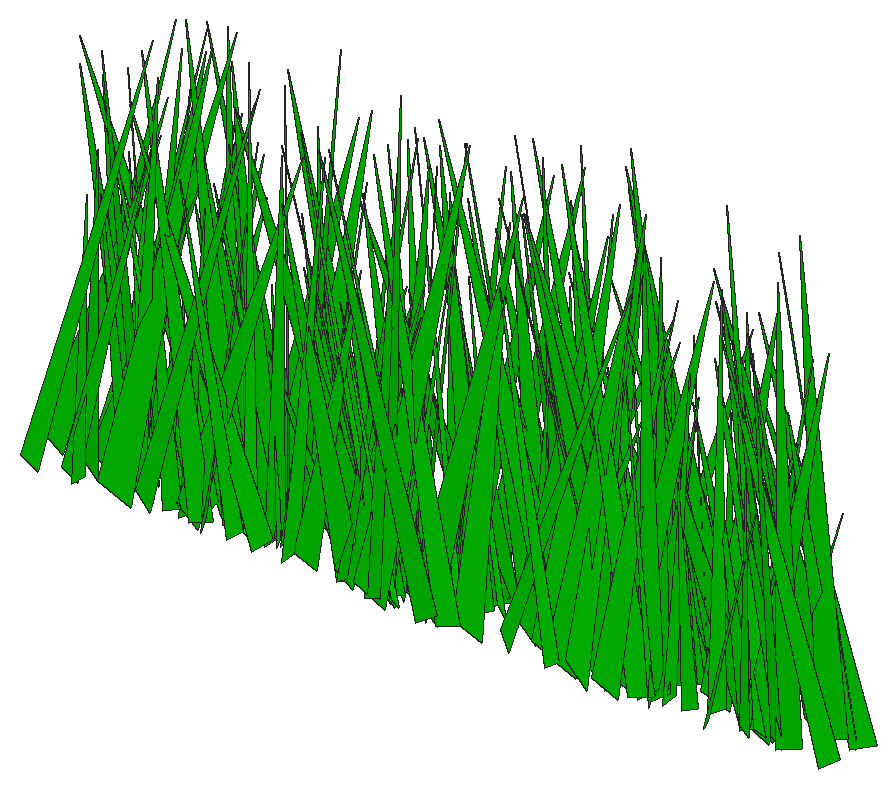
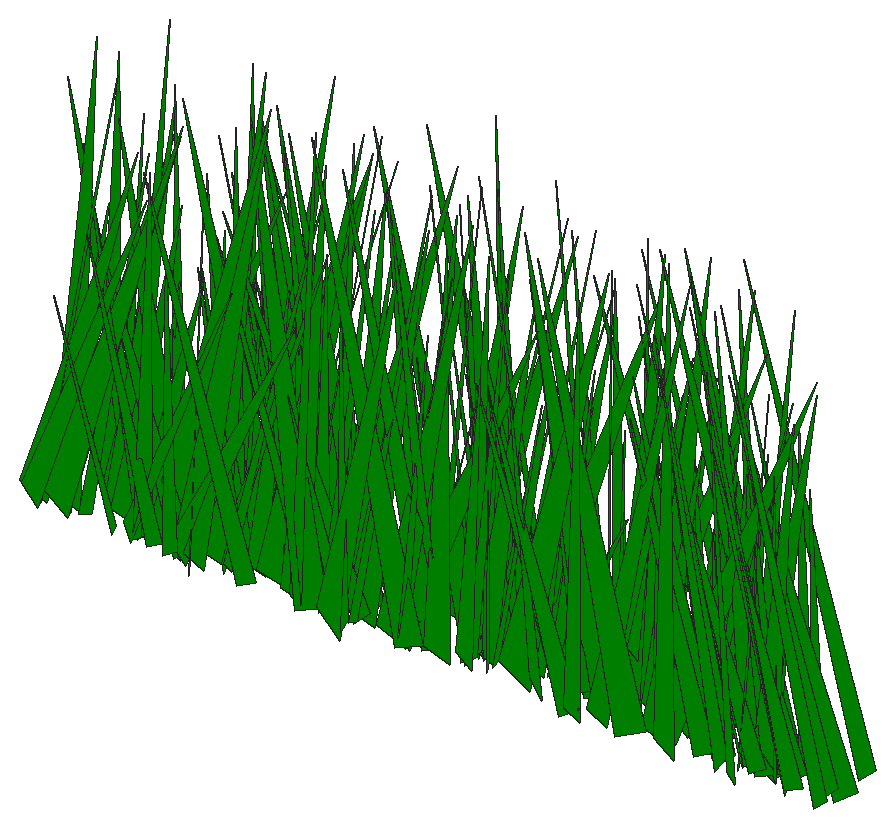
# SketchUp Ruby script. Lengths in inches.
U = 1.inch
M = Sketchup.active_model
def pt(a) = Geom::Point3d.new(a.map { |v| v * U })
def face(e, loops, mat)
  f = e.add_face(loops[0].map { |a| pt(a) })
  loops[1..].each { |l| e.add_face(l.map { |a| pt(a) }).erase! }
  f.material = f.back_material = mat if mat
  f
end
# faces: each face lists its corners as indices into pts; further lists are holes
def faces(e, pts, list, mat = nil) = list.each { |f| face(e, (f[0].is_a?(Array) ? f : [f]).map { |l| l.map { |i| pts[i] } }, mat) }
# xy, xz, yz: faces in a plane at the given z, y or x. An outline is a flat list of corners, or four numbers for a rectangle; further outlines are holes
def ring(l) = l.size == 4 ? [[l[0], l[1]], [l[2], l[1]], [l[2], l[3]], [l[0], l[3]]] : l.each_slice(2).to_a
def flat(e, list, mat, &to3) = list.each { |f| face(e, (f[0].is_a?(Array) ? f : [f]).map { |l| ring(l).map { |u, v| to3.(u, v) } }, mat) }
def xy(e, z, list, mat = nil) = flat(e, list, mat) { |x, y| [x, y, z] }
def xz(e, y, list, mat = nil) = flat(e, list, mat) { |x, z| [x, y, z] }
def yz(e, x, list, mat = nil) = flat(e, list, mat) { |y, z| [x, y, z] }
def lines(e, pts, list) = list.each { |a, b| e.add_line(pt(pts[a]), pt(pts[b])) }
# prism: a flat outline (further loops are holes) pulled along v
def prism(e, loops, v, mat = nil)
  f = face(e, loops, mat); d = Geom::Vector3d.new(v.map { |x| x * U })
  f.pushpull(f.normal.samedirection?(d) ? d.length : -d.length)
end
def box(e, o, s, mat = nil) = prism(e, [[o, [o[0] + s[0], o[1], o[2]], [o[0] + s[0], o[1] + s[1], o[2]], [o[0], o[1] + s[1], o[2]]]], [0, 0, s[2]], mat)
def at(x, y, z, deg = 0) = Geom::Transformation.translation(pt([x, y, z])) * Geom::Transformation.rotation(ORIGIN, Z_AXIS, deg.degrees)
def axes(o, x, y, z) = Geom::Transformation.new([*x, 0, *y, 0, *z, 0, *pt(o).to_a, 1])
def part(name) = M.definitions.add(name)
# library, detail: a bought-in or finely detailed component or shape, given as its bounding box
def library(name, o, s) = part(name).tap { |d| box(d.entities, o, s) }
def detail(e, o, s) = box(e.add_group.entities, o, s)
def put(e, d, t, mat = nil) = e.add_instance(d, t).tap { |i| i.material = mat if mat }
def group(e, t, mat = nil) = e.add_group.tap { |g| g.transformation = t; g.material = mat if mat }.entities
root = M.entities
M.materials.add("[Color G06]").color = [0, 204, 0]
c1 = part("fur_instance\#9")
p = [[0.8125,0,1.79],[0.67,-0.02,1.48],[0,-0.11,0],[0,0.11,0]]
faces(c1.entities,p,[[0,1,2,3]])
put(root,c1,axes([65.03,21.09,4.28],[2.52401,0.41304,0.13674],[2.69868,-0.32729,2.29658],[-1.22442,0.13009,5.34363]),"[Color G06]")
put(root,c1,axes([65.81,22.77,4.28],[1.4299,0.64828,0.60801],[4.40546,-0.20709,2.22153],[-1.53955,0.00952,6.92167]),"[Color G06]")
put(root,c1,axes([62.85,22.48,4.28],[1.91128,-0.58814,1.34913],[-4.02224,-0.19332,3.04702],[1.55738,0.22249,6.21382]),"[Color G06]")
put(root,c1,axes([63.18,23.32,4.28],[5.09653,0.36827,1.45993],[2.81479,-0.67384,-2.42358],[-0.07518,-0.26377,8.2296]),"[Color G06]")
put(root,c1,axes([66.39,22.39,4.28],[-1.18854,-0.59292,2.74747],[-4.56568,0.1052,-1.8038],[-0.78304,0.28655,6.34715]),"[Color G06]")
put(root,c1,axes([64.85,21.875,4.28],[-2.70554,-0.48129,0.88394],[-3.09665,0.3775,2.43972],[1.63501,-0.08146,6.08348]),"[Color G06]")
put(root,c1,axes([63.39,22.6,4.28],[4.15065,-0.36176,1.27161],[-2.72128,-0.53072,2.49719],[0.2207,0.25964,6.87607]),"[Color G06]")
put(root,c1,axes([65.39,22.8125,4.28],[3.17847,0.20749,1.96617],[1.21554,-0.477,1.39313],[-1.57071,0.05073,5.05684]),"[Color G06]")
put(root,c1,axes([66.02,22.18,4.28],[1.41975,0.39948,1.46758],[2.74012,-0.23385,1.3911],[-1.28956,-0.05708,4.57163]),"[Color G06]")
put(root,c1,axes([63.18,20.99,4.28],[5.58303,-0.32981,0.72359],[-2.41107,-0.75303,2.12599],[0.12329,0.20882,8.80923]),"[Color G06]")
put(root,c1,axes([64.39,23.09,4.28],[1.85161,0.50796,0.52107],[3.56109,-0.23758,-1.66117],[0.84239,-0.11219,5.87702]),"[Color G06]")
put(root,c1,axes([66.82,22.6875,4.28],[-4.87933,0.09071,1.77055],[0.15408,0.65216,-2.88967],[1.34269,0.2548,6.76579]),"[Color G06]")
put(root,c1,axes([64.625,21.18,4.28],[2.765,0.44984,0.6929],[3.24076,-0.37054,-1.25313],[0.34461,-0.12466,6.22514]),"[Color G06]")
put(root,c1,axes([65.6,22.35,4.28],[3.70495,-0.1304,2.29112],[-1.41871,-0.51302,1.77055],[-1.10075,0.22231,5.42958]),"[Color G06]")
put(root,c1,axes([67.02,22,4.28],[-4.04341,0.28436,0.34002],[1.71855,0.50764,-3.11833],[1.121,0.24743,6.00704]),"[Color G06]")
put(root,c1,axes([66.87,21.99,4.28],[-4.73597,-0.54642,0.1989],[-3.56902,0.61286,3.58328],[1.62315,-0.24675,8.45935]),"[Color G06]")
put(root,c1,axes([64.74,22.95,4.28],[5.91476,0.02042,1.22274],[-0.16214,-0.77575,3.24034],[-0.81515,0.30248,8.22767]),"[Color G06]")
put(root,c1,axes([69.79,22.69,4.28],[-3.88048,0.59537,0.1604],[3.94815,0.49235,3.42266],[-1.62873,-0.22498,7.9146]),"[Color G06]")
put(root,c1,axes([64.76,22.43,4.28],[3.01878,-0.43614,0.07582],[-2.99362,-0.39996,1.95415],[0.90724,0.13148,6.19585]),"[Color G06]")
put(root,c1,axes([68.56,21.85,4.28],[-4.66469,0.17717,0.03548],[1.2525,0.64312,-1.09291],[0.21482,0.09753,7.14258]),"[Color G06]")
put(root,c1,axes([66.32,23.72,4.28],[4.59361,-0.16988,1.65597],[-0.89452,-0.64182,-2.02099],[-1.38263,-0.14918,6.80925]),"[Color G06]")
put(root,c1,axes([66.26,22.77,4.28],[3.62073,0.46888,2.78339],[3.76191,-0.50551,-1.14876],[-0.78907,-0.2585,7.29518]),"[Color G06]")
put(root,c1,axes([65.74,22.38,4.28],[3.87765,0.01232,0.42972],[0.17029,-0.51726,-1.72892],[-0.24794,-0.16258,5.53311]),"[Color G06]")
put(root,c1,axes([65.48,22.8125,4.28],[0.91906,-0.84568,0.07059],[-5.8491,-0.12184,2.43318],[1.60285,0.04029,8.83863]),"[Color G06]")
put(root,c1,axes([66.81,21.61,4.28],[4.30907,-0.51266,0.59159],[-3.50288,-0.5931,-2.04957],[-1.18441,-0.11107,8.21388]),"[Color G06]")
put(root,c1,axes([65.125,22.53,4.28],[3.95646,0.65707,1.11878],[4.68493,-0.50937,-2.64232],[0.90289,-0.23627,8.80802]),"[Color G06]")
put(root,c1,axes([68.05,22.58,4.28],[-3.18293,-0.05703,1.34154],[-0.19512,0.45089,1.16793],[0.96691,-0.09676,4.65186]),"[Color G06]")
put(root,c1,axes([65.99,22.86,4.28],[2.42536,-0.38642,0.06063],[-2.65314,-0.32157,1.64142],[0.80098,0.10493,5.25344]),"[Color G06]")
put(root,c1,axes([68.39,21.47,4.28],[0.82399,0.49063,0.29271],[3.36067,-0.11785,1.55914],[-1.05997,0.00776,5.17088]),"[Color G06]")
put(root,c1,axes([66.43,21.1,4.28],[1.12716,0.85412,0.18448],[5.97781,-0.1495,-2.07028],[1.34081,-0.05147,9.07496]),"[Color G06]")
put(root,c1,axes([68.12,22.11,4.28],[-1.84068,0.27274,0.59621],[1.81979,0.26037,-1.13307],[0.82042,0.03438,3.85094]),"[Color G06]")
put(root,c1,axes([67.1,23.24,4.28],[4.3848,-0.15602,2.11483],[-1.59045,-0.57909,2.45812],[-0.85125,0.27829,6.30089]),"[Color G06]")
put(root,c1,axes([69.25,22.36,4.28],[-3.43614,0.13217,1.37215],[1.21555,0.456,1.75388],[0.51347,-0.19504,5.03036]),"[Color G06]")
put(root,c1,axes([69.5625,21.39,4.28],[-3.75264,0.50641,2.32915],[3.92827,0.5107,1.382],[0.43111,-0.24543,7.68156]),"[Color G06]")
put(root,c1,axes([67.34,22.8125,4.28],[2.1187,0.58009,2.12969],[4.36515,-0.25086,-1.85098],[0.53032,-0.25266,6.72731]),"[Color G06]")
put(root,c1,axes([66.64,22.8,4.28],[5.66602,0.00721,0.28285],[0.08859,-0.77449,-1.69551],[-0.17505,-0.15851,8.29716]),"[Color G06]")
put(root,c1,axes([68.92,21.46,4.28],[2.70661,0.42818,0.19516],[2.88812,-0.36265,1.92962],[-1.05097,0.10615,5.80533]),"[Color G06]")
put(root,c1,axes([69.91,23.0625,4.28],[0.07231,-0.53144,0.33611],[-3.70129,-0.01745,-1.38995],[-0.93558,0.02794,5.5248]),"[Color G06]")
put(root,c1,axes([69.0625,23.57,4.28],[4.93503,-0.46453,1.81542],[-2.88141,-0.69456,-2.9194],[-2.06642,-0.14089,8.40639]),"[Color G06]")
put(root,c1,axes([67.87,23.07,4.28],[0.82857,0.54581,0.87456],[3.78653,-0.08508,-1.91352],[1.15107,-0.113,5.66515]),"[Color G06]")
put(root,c1,axes([67.97,22.73,4.28],[0.05659,0.66927,0.063],[4.59026,-0.00583,-2.09684],[1.40245,-0.00793,6.86047]),"[Color G06]")
put(root,c1,axes([71.9375,21.4,4.28],[-4.14515,0.46374,0.31304],[3.17829,0.53623,2.75445],[-1.00096,-0.21775,7.44971]),"[Color G06]")
put(root,c1,axes([70.625,21.92,4.28],[-2.07026,0.74776,1.89532],[5.50104,0.26954,1.20622],[-0.3188,-0.20484,8.50589]),"[Color G06]")
put(root,c1,axes([67.37,21.3,4.28],[4.80707,0.42204,0.91107],[3.07434,-0.63993,-2.1802],[0.28313,-0.2169,8.20522]),"[Color G06]")
put(root,c1,axes([70.89,21.37,4.28],[-3.46219,0.27787,2.20599],[2.42843,0.45149,1.98048],[0.50212,-0.26759,5.63232]),"[Color G06]")
put(root,c1,axes([71.82,23.37,4.28],[-4.18526,-0.55616,1.17124],[-4.06422,0.57046,-1.32345],[-0.05584,0.16471,8.53861]),"[Color G06]")
put(root,c1,axes([70.09,22.71,4.28],[3.01449,-0.11,1.79283],[-0.52411,-0.44649,-1.17833],[-1.33659,-0.073,4.50554]),"[Color G06]")
put(root,c1,axes([69.73,21.29,4.28],[4.92092,0.26688,0.96305],[1.49677,-0.64089,3.31846],[-1.35565,0.26115,7.15969]),"[Color G06]")
put(root,c1,axes([71.8,21.92,4.28],[-0.78227,-0.62233,0.99126],[-4.41584,0.08634,-1.55762],[-0.92603,0.11401,6.59023]),"[Color G06]")
put(root,c1,axes([72.38,22.14,4.28],[-3.76174,0.24185,0.92044],[1.83675,0.50574,1.50268],[0.11696,-0.1636,6.00585]),"[Color G06]")
put(root,c1,axes([72.05,21.97,4.28],[-1.56858,0.5856,1.46351],[4.29231,0.19812,1.16949],[-0.41294,-0.16503,6.5971]),"[Color G06]")
put(root,c1,axes([71.875,22,4.28],[1.55614,-0.66248,3.53345],[-5.0686,-0.28729,-1.2013],[-1.57129,0.27063,7.37444]),"[Color G06]")
put(root,c1,axes([69.01,21.43,4.28],[3.32263,0.56403,1.15313],[3.99903,-0.40905,-2.75526],[0.98154,-0.24275,7.32215]),"[Color G06]")
put(root,c1,axes([71.45,21.45,4.28],[-5.06818,0.304,2.53352],[1.81394,0.73898,-2.08072],[2.0823,0.09618,7.97899]),"[Color G06]")
put(root,c1,axes([71.09,22.93,4.28],[1.0439,0.48006,0.89698],[3.438,-0.12543,-1.22591],[0.62623,-0.11163,5.235]),"[Color G06]")
put(root,c1,axes([72.47,22.07,4.28],[-5.37227,0.02684,3.25162],[-0.82329,0.72123,-3.72224],[2.02301,0.36479,7.12015]),"[Color G06]")
put(root,c1,axes([72.19,21.89,4.28],[2.99065,-0.10963,1.74873],[-0.37245,-0.43053,-1.67761],[-1.35953,-0.1232,4.30637]),"[Color G06]")
put(root,c1,axes([70.43,23.48,4.28],[1.30926,-0.76074,0.9804],[-5.25919,-0.14625,2.65162],[1.59171,0.14251,7.95483]),"[Color G06]")
put(root,c1,axes([72,21.93,4.28],[4.21841,-0.48531,0.41862],[-3.18381,-0.55981,-2.88768],[-1.43332,-0.18484,7.6464]),"[Color G06]")
put(root,c1,axes([72.56,23.68,4.28],[3.96034,-0.38082,1.9523],[-2.4548,-0.5795,-1.86191],[-1.77151,-0.04831,6.94459]),"[Color G06]")
put(root,c1,axes([72.3125,21.92,4.28],[3.20505,-0.06638,0.79692],[-0.35441,-0.44422,-1.06677],[-0.62074,-0.08912,4.72377]),"[Color G06]")
put(root,c1,axes([75.68,22.1,4.28],[-2.05281,-0.73205,1.07105],[-4.92219,0.22382,-3.49963],[-1.96091,0.20453,7.66335]),"[Color G06]")
put(root,c1,axes([74.79,21.97,4.28],[-1.22953,-0.3178,1.13811],[-2.09707,0.08368,-2.37622],[-1.17311,0.18349,3.05493]),"[Color G06]")
put(root,c1,axes([75.43,22.9,4.28],[-0.80993,0.79684,1.37115],[5.47842,0.06391,2.9622],[-1.86608,-0.15823,8.10129]),"[Color G06]")
put(root,c1,axes([72.79,22.15,4.28],[5.42873,0.35696,2.16338],[2.37533,-0.7821,1.50985],[-1.73377,0.04621,8.84246]),"[Color G06]")
put(root,c1,axes([74.57,21.99,4.28],[-3.76647,0.27592,0.38001],[1.88209,0.51657,-1.41851],[0.66161,0.1013,6.19857]),"[Color G06]")
put(root,c1,axes([72.5625,22.27,4.28],[0.0275,0.82204,0.34043],[5.73797,0.00365,-2.04921],[1.37107,-0.03178,8.56915]),"[Color G06]")
put(root,c1,axes([73.16,22.35,4.28],[-2.10897,0.29137,2.49274],[2.02983,0.3673,-1.09584],[1.74001,-0.07531,4.29967]),"[Color G06]")
put(root,c1,axes([73.01,21.41,4.28],[4.86811,-0.37541,0.71689],[-2.46528,-0.6616,-2.40467],[-1.18334,-0.16608,7.95889]),"[Color G06]")
put(root,c1,axes([75.36,22.08,4.28],[-0.83923,0.44019,2.06664],[3.32258,0.05065,1.77448],[-0.91503,-0.21979,4.54789]),"[Color G06]")
put(root,c1,axes([75.375,21.4,4.28],[-0.20066,-0.67545,0.01455],[-4.70252,0.02684,-1.738],[-1.16149,0.00803,7.03414]),"[Color G06]")
put(root,c1,axes([72.7,23.64,4.28],[1.04211,-0.51377,0.16453],[-3.4227,-0.12896,2.16717],[1.36813,0.06873,5.29635]),"[Color G06]")
put(root,c1,axes([75.19,22.21,4.28],[-0.30905,0.4476,0.98193],[3.18286,0.01918,1.23341],[-0.77747,-0.09941,4.65911]),"[Color G06]")
put(root,c1,axes([73.52,21.86,4.28],[4.50254,0.24071,1.08624],[1.58137,-0.62997,1.3947],[-1.00362,0.08728,7.07074]),"[Color G06]")
put(root,c1,axes([76.82,21.38,4.28],[-5.31766,-0.09753,0.2792],[-0.72377,0.71225,-2.21115],[-0.01501,0.20793,7.70509]),"[Color G06]")
put(root,c1,axes([74.4,23.11,4.28],[3.34188,0.37288,0.21425],[2.39419,-0.43036,2.6238],[-1.19951,0.17986,5.83393]),"[Color G06]")
put(root,c1,axes([73.57,21.46,4.28],[1.11263,-0.5672,0.19002],[-3.97672,-0.14764,1.38899],[0.86411,0.05089,6.1476]),"[Color G06]")
put(root,c1,axes([73.12,23.26,4.28],[3.1082,-0.31117,0.51872],[-2.19761,-0.39781,2.00115],[0.51996,0.17873,5.35707]),"[Color G06]")
put(root,c1,axes([76.48,21.57,4.28],[-5.70657,-0.07445,1.44317],[-0.1169,0.7461,3.38877],[1.09716,-0.30772,7.86733]),"[Color G06]")
put(root,c1,axes([76.34,22.65,4.28],[-3.53979,0.10199,0.4973],[0.64484,0.48563,-1.18796],[0.47939,0.09985,5.26999]),"[Color G06]")
put(root,c1,axes([75.23,22.63,4.28],[2.5036,-0.24634,0.04899],[-1.64316,-0.32754,-1.61847],[-0.64941,-0.12092,4.28397]),"[Color G06]")
put(root,c1,axes([76.98,22.51,4.28],[-0.81022,0.58999,1.94612],[4.35299,0.07262,1.51916],[-0.80493,-0.20115,6.25657]),"[Color G06]")
put(root,c1,axes([76.99,21.53,4.28],[-0.70741,0.50007,0.45916],[3.49655,0.08512,1.38325],[-0.8537,-0.06573,5.28499]),"[Color G06]")
put(root,c1,axes([77.33,21.125,4.28],[-3.54295,0.12044,0.09276],[0.82512,0.4806,-1.28852],[0.26282,0.11482,5.29579]),"[Color G06]")
put(root,c1,axes([77.05,22.99,4.28],[-4.78468,0.25107,1.21329],[1.59675,0.66635,-1.77467],[1.16244,0.11813,7.43166]),"[Color G06]")
put(root,c1,axes([76.41,22.96,4.28],[2.77754,0.05368,1.99231],[-0.07473,-0.40956,1.50037],[-1.38549,0.1297,3.91315]),"[Color G06]")
put(root,c1,axes([74.79,21.59,4.28],[3.76624,0.09429,0.01742],[0.66587,-0.51541,-1.09519],[0.11823,-0.10086,5.61307]),"[Color G06]")
put(root,c1,axes([75.14,21.26,4.28],[5.30632,0.34491,0.846],[2.35078,-0.73712,1.5863],[-0.95506,0.10198,8.60496]),"[Color G06]")
put(root,c1,axes([76.7,22.17,4.28],[-2.63992,0.29473,0.74874],[1.93653,0.36915,-1.44087],[0.98396,0.06424,4.84461]),"[Color G06]")
put(root,c1,axes([78.65,20.98,4.28],[-3.6349,-0.55348,1.58477],[-4.04953,0.4494,-2.71751],[-0.69267,0.27716,7.57095]),"[Color G06]")
put(root,c1,axes([77.18,22.77,4.28],[-4.42167,0.47999,0.52294],[3.19709,0.59709,-2.57387],[1.32268,0.16134,7.96957]),"[Color G06]")
put(root,c1,axes([78.3,21.43,4.28],[-5.85793,-0.10273,0.87864],[-0.44298,0.75561,3.55116],[0.8319,-0.321,8.07795]),"[Color G06]")
put(root,c1,axes([77.19,23.12,4.28],[1.82483,0.45762,0.97878],[3.06297,-0.2703,1.76175],[-1.34793,0.00531,5.32839]),"[Color G06]")
put(root,c1,axes([75.17,21.34,4.28],[2.44703,0.46136,1.08856],[3.32692,-0.30363,-1.92288],[0.63908,-0.1859,5.84205]),"[Color G06]")
put(root,c1,axes([76.57,20.97,4.28],[4.2427,0.44603,1.91021],[3.09923,-0.61771,1.19259],[-1.50305,-0.01469,7.85109]),"[Color G06]")
put(root,c1,axes([79.79,23.08,4.28],[-2.11587,-0.63042,0.86213],[-4.09341,0.22388,-3.63492],[-2.0039,0.20834,6.51483]),"[Color G06]")
put(root,c1,axes([76.9375,21.28,4.28],[-4.77018,-0.45541,3.43123],[-3.03774,0.73773,1.81456],[2.59009,0.02651,8.44749]),"[Color G06]")
put(root,c1,axes([76.47,22.26,4.28],[-2.09382,-0.72398,1.25228],[-4.90204,0.31422,2.55998],[1.90458,0.01283,7.96562]),"[Color G06]")
put(root,c1,axes([76.99,22.47,4.28],[-4.59396,-0.13413,3.85846],[-0.29696,0.71999,2.08544],[2.73897,-0.14691,6.69774]),"[Color G06]")
put(root,c1,axes([76.9375,21.26,4.28],[3.11936,-0.06098,1.23534],[-0.71632,-0.41385,1.69346],[-0.60111,0.1767,4.39258]),"[Color G06]")
put(root,c1,axes([77.04,21.78,4.28],[4.24261,-0.00725,1.82871],[-0.59335,-0.55035,2.82437],[-1.07133,0.27611,5.67767]),"[Color G06]")
put(root,c1,axes([79.43,21.0625,4.28],[-3.76977,0.53782,1.26296],[3.94824,0.51474,1.14406],[0.03059,-0.15894,7.97893]),"[Color G06]")
put(root,c1,axes([77.29,22.4,4.28],[5.21289,0.21658,1.92074],[1.3298,-0.74286,1.56071],[-1.51511,0.09318,7.9783]),"[Color G06]")
put(root,c1,axes([79.27,22.81,4.28],[-3.97242,-0.12414,0.23598],[-0.76446,0.51414,2.32441],[0.48273,-0.20733,5.62283]),"[Color G06]")
put(root,c1,axes([78.07,23.36,4.28],[2.66797,-0.61267,0.59516],[-4.25331,-0.37445,-1.69029],[-1.1712,-0.0358,7.49418]),"[Color G06]")
put(root,c1,axes([76.41,21.02,4.28],[2.07971,0.79011,1.57005],[5.65403,-0.24968,-2.29568],[1.11357,-0.2079,8.72381]),"[Color G06]")
put(root,c1,axes([79.47,21.59,4.28],[-5.77122,0.18187,1.5232],[0.90161,0.77772,-3.03657],[1.38809,0.25099,8.30532]),"[Color G06]")
put(root,c1,axes([79.94,23.29,4.28],[-2.13821,-0.69489,1.31662],[-5.00859,0.27155,-1.70551],[-0.72283,0.17393,7.92296]),"[Color G06]")
put(root,c1,axes([79.74,22.25,4.28],[1.99161,0.75447,0.98433],[5.04107,-0.29216,2.94087],[-2.07243,0.01439,8.09946]),"[Color G06]")
put(root,c1,axes([80.19,22.76,4.28],[-5.01233,0.14907,0.66192],[0.84433,0.65891,-2.76477],[0.79124,0.24121,7.14341]),"[Color G06]")
put(root,c1,axes([79.36,23.44,4.28],[3.15869,-0.2092,2.42452],[-1.15395,-0.49273,-1.52587],[-1.88434,-0.04894,4.99862]),"[Color G06]")
put(root,c1,axes([78.32,23.06,4.28],[4.15436,0.52324,0.48951],[3.57984,-0.56965,2.08288],[-1.17113,0.11482,8.1033]),"[Color G06]")
put(root,c1,axes([78.86,22.01,4.28],[3.08871,0.02712,1.19388],[0.38308,-0.43064,-1.0901],[-0.72744,-0.11164,4.49516]),"[Color G06]")
put(root,c1,axes([81.34,23.34,4.28],[-5.23885,-0.29845,0.87176],[-2.05221,0.73125,1.20993],[0.8422,-0.07461,8.37106]),"[Color G06]")
put(root,c1,axes([78.37,23.14,4.28],[3.41493,0.60149,1.5499],[4.41942,-0.44531,-1.89848],[0.38715,-0.2222,8.00037]),"[Color G06]")
put(root,c1,axes([81.38,22.94,4.28],[-0.71484,-0.71068,0.76758],[-5.02724,0.08348,-1.57956],[-0.982,0.08998,7.52763]),"[Color G06]")
put(root,c1,axes([78.28,21.38,4.28],[-1.45228,-0.74366,3.15273],[-4.92383,0.31726,3.53022],[2.94047,0.16396,7.46848]),"[Color G06]")
put(root,c1,axes([82.95,22.23,4.28],[-3.98797,0.65238,1.04512],[4.63968,0.5146,2.64613],[-0.92167,-0.23226,8.79851]),"[Color G06]")
put(root,c1,axes([80.1,21.18,4.28],[-1.54131,0.71998,0.54111],[4.99147,0.2207,-1.97466],[1.36927,0.00592,7.80743]),"[Color G06]")
put(root,c1,axes([81.89,23.87,4.28],[2.98312,-0.63805,0.66019],[-3.81905,-0.38486,-4.18157],[-2.55857,-0.16945,7.01136]),"[Color G06]")
put(root,c1,axes([79.08,23.46,4.28],[3.63512,-0.64812,0.99468],[-4.66317,-0.48465,1.7904],[0.54813,0.17514,8.63519]),"[Color G06]")
put(root,c1,axes([81.96,22.69,4.28],[0.23917,0.75006,1.32153],[5.34869,-0.0561,1.49553],[-1.05164,-0.11475,7.90691]),"[Color G06]")
put(root,c1,axes([82.76,22.91,4.28],[-1.66817,-0.3698,0.88602],[-2.65824,0.20194,-1.49731],[-0.56398,0.142,4.43665]),"[Color G06]")
put(root,c1,axes([81.34,23.85,4.28],[-3.4163,-0.40056,0.86724],[-2.22926,0.43588,3.51099],[1.90218,-0.20856,5.67225]),"[Color G06]")
put(root,c1,axes([82.52,23.26,4.28],[-4.50022,-0.39536,0.70533],[-2.6082,0.6131,2.30549],[1.20763,-0.14914,7.60778]),"[Color G06]")
put(root,c1,axes([81.39,22.76,4.28],[2.87235,-0.25457,0.46337],[-1.67908,-0.39171,-1.47127],[-0.78069,-0.09413,4.8692]),"[Color G06]")
put(root,c1,axes([82.49,22.65,4.28],[4.31574,0.37946,3.4976],[2.67636,-0.6803,1.10174],[-2.39134,-0.07656,7.54531]),"[Color G06]")
put(root,c1,axes([84.15,22.33,4.28],[-6.04732,0.03996,1.22018],[0.11794,0.83435,-1.83333],[0.85717,0.16713,8.86063]),"[Color G06]")
put(root,c1,axes([83.4375,21.12,4.28],[-3.86873,0.24433,1.83568],[2.02314,0.5329,1.37624],[0.69676,-0.19074,6.19648]),"[Color G06]")
put(root,c1,axes([81.73,23.42,4.28],[0.37525,-0.37242,0.47545],[-2.4647,-0.02968,1.67425],[1.07675,0.06185,3.66669]),"[Color G06]")
put(root,c1,axes([83.25,22.55,4.28],[-2.96065,0.4347,1.04331],[3.01752,0.42411,-1.17174],[1.04858,0.00687,6.31773]),"[Color G06]")
put(root,c1,axes([83.55,23.4,4.28],[-4.91565,-0.28049,3.33792],[-2.47244,0.71683,-1.21357],[1.7091,0.23024,7.84479]),"[Color G06]")
put(root,c1,axes([85.05,22.74,4.28],[-4.4211,0.57114,1.103],[4.16064,0.6031,1.37753],[-0.09605,-0.1641,8.90145]),"[Color G06]")
put(root,c1,axes([81.39,22.35,4.28],[-2.01232,-0.69572,2.70708],[-4.43572,0.36877,3.52186],[2.91498,0.08088,7.22803]),"[Color G06]")
put(root,c1,axes([83.71,23.18,4.28],[1.2238,-0.69849,1.93697],[-5.06155,-0.20013,-1.14721],[-1.073,0.14741,7.62078]),"[Color G06]")
put(root,c1,axes([85.66,21.71,4.28],[-5.75347,-0.06776,0.01608],[-0.47983,0.79468,1.18738],[0.07748,-0.11027,8.54752]),"[Color G06]")
put(root,c1,axes([84.27,22.2,4.28],[1.02378,-0.40725,1.37736],[-2.7598,-0.18142,-1.57992],[-1.32741,0.0631,4.3471]),"[Color G06]")
put(root,c1,axes([83.31,23.07,4.28],[-1.46691,-0.53691,0.07384],[-3.66878,0.19712,1.84324],[1.16934,-0.05509,5.87573]),"[Color G06]")
put(root,c1,axes([83.28,22.36,4.28],[-4.3401,0.39894,2.90939],[2.2587,0.65648,-2.81422],[2.62151,0.09484,7.24145]),"[Color G06]")
put(root,c1,axes([85.625,21.79,4.28],[-1.5185,-0.76189,0.60774],[-5.33722,0.19241,-2.07823],[-1.23761,0.10502,8.21669]),"[Color G06]")
put(root,c1,axes([81.38,21.39,4.28],[5.0585,0.28199,0.17883],[1.95284,-0.66687,-2.59215],[0.53864,-0.2305,7.7184]),"[Color G06]")
put(root,c1,axes([83.37,22.13,4.28],[-0.17996,-0.48456,0.91126],[-3.44966,0.042,1.04404],[0.73914,0.07806,5.09454]),"[Color G06]")
put(root,c1,axes([81.29,22.98,4.28],[3.43961,0.50773,0.07671],[3.35007,-0.43736,-3.00067],[1.42725,-0.19703,6.85835]),"[Color G06]")
put(root,c1,axes([82.95,21.57,4.28],[-1.1244,0.84264,0.49647],[5.78886,0.16349,-2.59058],[1.76486,0.00059,8.81357]),"[Color G06]")
put(root,c1,axes([84.06,22.05,4.28],[2.12729,-0.2889,0.08187],[-1.93976,-0.2814,-1.48366],[-0.7297,-0.09416,4.18268]),"[Color G06]")
put(root,c1,axes([82.84,23.48,4.28],[-0.04771,-0.85231,0.09227],[-5.88274,0.00874,2.48026],[1.66001,0.00648,8.7922]),"[Color G06]")
put(root,c1,axes([86.95,21.83,4.28],[-3.0093,-0.69653,0.13584],[-4.81254,0.4002,-2.41802],[-1.34091,0.12687,8.37344]),"[Color G06]")
put(root,c1,axes([86.4375,23.06,4.28],[-5.14387,0.12512,0.6686],[0.96138,0.70807,1.29994],[0.28453,-0.13049,7.69495]),"[Color G06]")
put(root,c1,axes([86.84,22.84,4.28],[-4.89689,-0.15802,0.40527],[-1.13481,0.60976,-3.31794],[-0.2642,0.30968,6.73972]),"[Color G06]")
put(root,c1,axes([82.92,21.625,4.28],[2.52204,-0.37612,0.38833],[-2.55898,-0.31431,2.15271],[0.89128,0.16188,5.08184]),"[Color G06]")
put(root,c1,axes([84.01,22.68,4.28],[-2.11933,0.50953,3.16635],[3.78084,0.3762,-1.30167],[1.88291,-0.18189,6.17764]),"[Color G06]")
put(root,c1,axes([83.02,23.22,4.28],[3.49931,0.35606,0.37771],[2.51984,-0.46564,-1.72272],[0.48379,-0.15009,6.24087]),"[Color G06]")
put(root,c1,axes([85.65,22.66,4.28],[1.23889,-0.41855,2.03364],[-3.06519,-0.2208,-1.04921],[-1.21044,0.13075,4.73833]),"[Color G06]")
put(root,c1,axes([83.7,21.24,4.28],[0.15552,0.71235,2.63984],[5.18796,0.04948,-2.2165],[1.51694,-0.24225,7.30983]),"[Color G06]")
put(root,c1,axes([86.79,21.28,4.28],[3.01773,-0.53302,5.62265],[-4.34468,-0.59588,-1.28042],[-3.14447,0.31179,7.16518]),"[Color G06]")
put(root,c1,axes([84.41,21.1,4.28],[-3.97025,0.5706,1.99514],[3.27809,0.56497,-3.99011],[2.78925,0.14821,7.52932]),"[Color G06]")
put(root,c1,axes([84.68,21.6,4.28],[-0.61937,-0.4776,1.76222],[-3.48869,0.12354,1.10726],[0.97473,0.13867,5.08277]),"[Color G06]")
put(root,c1,axes([88.2,23.31,4.28],[-2.24592,0.44644,0.7925],[2.8698,0.23126,3.20165],[-1.51497,-0.22376,4.88999]),"[Color G06]")
put(root,c1,axes([86.63,22.18,4.28],[-3.63483,0.09483,1.31076],[0.44235,0.50789,-1.48104],[1.01782,0.11793,5.32465]),"[Color G06]")
put(root,c1,axes([87.35,22.85,4.28],[-2.01213,0.77947,2.56364],[5.83324,0.25025,1.4862],[-0.40108,-0.27076,8.75381]),"[Color G06]")
put(root,c1,axes([87.78,23.3,4.28],[-0.38626,-0.70874,3.78066],[-5.45361,-0.05194,-2.36309],[-1.5778,0.35303,7.2424]),"[Color G06]")
put(root,c1,axes([85.59,21.07,4.28],[3.32077,0.15572,0.71963],[0.95257,-0.45445,1.478],[-0.75599,0.1114,5.02333]),"[Color G06]")
put(root,c1,axes([85.1,21.34,4.28],[5.08423,-0.03006,1.3312],[-0.48837,-0.68135,2.39883],[-0.77544,0.23201,7.21738]),"[Color G06]")
put(root,c1,axes([85.6,20.99,4.28],[-0.57122,0.65515,0.60856],[4.51875,0.0924,-1.95298],[1.34919,-0.0321,6.79865]),"[Color G06]")
put(root,c1,axes([88.84,23.16,4.28],[-1.22543,0.81333,2.32816],[5.74541,0.08906,3.18092],[-1.85364,-0.26163,8.32024]),"[Color G06]")
put(root,c1,axes([87.08,21.38,4.28],[-3.88876,-0.05148,2.10166],[0.27402,0.52396,2.60695],[1.4278,-0.24077,5.22379]),"[Color G06]")
put(root,c1,axes([86.12,22.92,4.28],[2.54291,-0.30267,1.55114],[-2.38947,-0.34226,1.07836],[-0.28032,0.17187,4.879]),"[Color G06]")
put(root,c1,axes([87.28,21.61,4.28],[3.66098,0.57842,1.21065],[3.75155,-0.51357,2.84608],[-1.94621,0.09808,7.76348]),"[Color G06]")
put(root,c1,axes([86.16,22.56,4.28],[0.41332,-0.46687,1.07314],[-3.32079,-0.03005,1.35499],[0.83519,0.11155,4.85645]),"[Color G06]")
put(root,c1,axes([86.9,21.61,4.28],[4.31562,-0.6295,0.63495],[-4.17964,-0.58399,-3.05409],[-1.75791,-0.1569,8.82027]),"[Color G06]")
put(root,c1,axes([87.37,22.71,4.28],[1.66536,-0.52749,0.33864],[-3.693,-0.23365,-1.23994],[-0.84988,-0.01836,6.05151]),"[Color G06]")
put(root,c1,axes([87.36,23.78,4.28],[-4.18178,-0.18956,2.10226],[-0.5869,0.56318,3.22578],[1.86602,-0.24768,5.72578]),"[Color G06]")
put(root,c1,axes([85.75,21.56,4.28],[1.18358,0.76091,0.62674],[5.31585,-0.14561,-2.11567],[1.30131,-0.09724,8.07247]),"[Color G06]")
put(root,c1,axes([85.36,23.53,4.28],[3.85989,-0.41585,0.00665],[-2.93309,-0.5292,1.32543],[0.53873,0.09823,7.16858]),"[Color G06]")
put(root,c1,axes([90.1875,22.28,4.28],[-3.61776,-0.54017,1.17884],[-3.69158,0.40828,-3.81502],[-1.41426,0.31607,6.94266]),"[Color G06]")
put(root,c1,axes([88.7,22.93,4.28],[-0.94093,-0.47768,1.19383],[-3.41057,0.09569,-1.60615],[-0.86049,0.14306,5.06059]),"[Color G06]")
put(root,c1,axes([90.2,23.26,4.28],[-3.59956,-0.25472,0.04806],[-1.67715,0.45679,-2.47903],[-0.72449,0.20811,5.50001]),"[Color G06]")
put(root,c1,axes([87.61,21.625,4.28],[3.89066,-0.30992,0.76438],[-1.99789,-0.53118,-2.02536],[-1.09983,-0.13143,6.38315]),"[Color G06]")
put(root,c1,axes([88.4375,21.58,4.28],[1.42223,-0.37232,0.23105],[-2.56871,-0.19696,-1.14035],[-0.74462,-0.03167,4.37515]),"[Color G06]")
put(root,c1,axes([88.37,23.47,4.28],[-2.15956,-0.40501,0.83362],[-2.68083,0.30874,1.71828],[1.24906,-0.0376,5.1292]),"[Color G06]")
put(root,c1,axes([90.05,22.72,4.28],[-0.56203,0.5143,0.43654],[3.49065,0.06006,1.91039],[-1.22615,-0.06476,5.23844]),"[Color G06]")
put(root,c1,axes([89.63,23.22,4.28],[-3.49288,0.43857,1.08201],[2.98515,0.49557,-1.54961],[1.22671,0.04282,6.85177]),"[Color G06]")
put(root,c1,axes([89.17,22,4.28],[4.31761,-0.39765,1.93047],[-2.6349,-0.62729,-1.67981],[-1.69049,-0.0379,7.5488]),"[Color G06]")
put(root,c1,axes([88.69,22.5,4.28],[0.34712,0.72906,0.44108],[5.144,-0.03975,-1.4948],[0.98034,-0.04956,7.68724]),"[Color G06]")
put(root,c1,axes([90.98,22.57,4.28],[-2.24623,0.49663,0.86424],[3.5882,0.29751,1.1925],[-0.37832,-0.12688,6.1791]),"[Color G06]")
put(root,c1,axes([87.99,23.25,4.28],[0.88328,-0.52424,0.48066],[-3.43143,-0.09245,2.5023],[1.56924,0.09292,5.20121]),"[Color G06]")
put(root,c1,axes([90.59,21.72,4.28],[0.58798,0.40364,1.14768],[2.81207,-0.11195,1.3047],[-1.02996,-0.07521,4.21739]),"[Color G06]")
put(root,c1,axes([89.43,21.13,4.28],[2.94253,0.13884,0.10645],[0.91681,-0.38813,1.54378],[-0.39478,0.13347,4.37859]),"[Color G06]")
put(root,c1,axes([91.2,22.38,4.28],[0.29684,-0.73074,1.07017],[-5.1646,-0.06161,-1.63282],[-1.14046,0.08881,7.6728]),"[Color G06]")
put(root,c1,axes([91.18,21.73,4.28],[-5.39388,0.42056,1.67045],[2.86136,0.76641,-1.52727],[1.46891,0.05138,9.109]),"[Color G06]")
put(root,c1,axes([89.04,23.38,4.28],[2.80414,-0.3175,0.56081],[-2.29762,-0.37649,1.1764],[0.21453,0.11786,5.26886]),"[Color G06]")
put(root,c1,axes([93.08,23.2,4.28],[-2.36074,-0.70653,1.0013],[-4.84328,0.27641,-3.10186],[-1.63198,0.20173,7.75706]),"[Color G06]")
put(root,c1,axes([90.58,21.55,4.28],[-2.38002,-0.28875,1.44512],[-1.9374,0.35818,1.09413],[1.21213,0.00553,4.58628]),"[Color G06]")
put(root,c1,axes([92.85,22.74,4.28],[-5.25523,0.05385,0.26865],[0.4167,0.71421,1.76373],[0.08819,-0.166,7.67547]),"[Color G06]")
put(root,c1,axes([89.67,23.24,4.28],[4.16513,0.21699,1.57404],[1.78884,-0.56722,-1.59082],[-0.57506,-0.19279,6.45213]),"[Color G06]")
put(root,c1,axes([91.52,22.12,4.28],[-4.06258,-0.46433,0.20501],[-3.14287,0.54382,2.3746],[1.10863,-0.15985,7.48305]),"[Color G06]")
put(root,c1,axes([91.91,23.15,4.28],[-3.96792,-0.39488,0.29459],[-2.76905,0.54884,1.19911],[0.6247,-0.07539,7.18636]),"[Color G06]")
put(root,c1,axes([92.01,21.79,4.28],[-0.08792,-0.44993,0.3723],[-3.11989,0.00255,-1.29134],[-0.85973,0.03675,4.64811]),"[Color G06]")
put(root,c1,axes([91.77,21.65,4.28],[-3.85602,-0.34868,1.64643],[-2.36742,0.559,1.21438],[1.36432,-0.0155,6.76057]),"[Color G06]")
put(root,c1,axes([93.94,23.32,4.28],[-3.1,-0.47989,0.53524],[-3.27402,0.38516,-2.6873],[-1.11904,0.20251,6.37961]),"[Color G06]")
put(root,c1,axes([90.6,23.41,4.28],[2.83821,-0.04522,0.25586],[-0.361,-0.37729,1.28472],[-0.06445,0.12189,4.07163]),"[Color G06]")
put(root,c1,axes([93.85,21.6,4.28],[-3.77275,0.45443,0.89614],[3.2575,0.48545,2.35473],[-0.60681,-0.21931,7.06909]),"[Color G06]")
put(root,c1,axes([94.02,23.04,4.28],[-2.47641,0.64523,0.01672],[4.44234,0.33103,2.20325],[-1.29467,-0.09832,7.52794]),"[Color G06]")
put(root,c1,axes([92.3125,21.55,4.28],[2.44034,0.70588,1.40088],[4.901,-0.36282,1.93065],[-1.57582,-0.03528,8.17398]),"[Color G06]")
put(root,c1,axes([92.92,23.15,4.28],[0.86499,-0.53886,0.90469],[-3.69192,-0.14103,-1.76478],[-1.29187,0.04224,5.64916]),"[Color G06]")
put(root,c1,axes([93.75,23.04,4.28],[-5.69539,-0.05766,1.34369],[-0.63058,0.77586,-2.14603],[0.76263,0.21095,8.26036]),"[Color G06]")
put(root,c1,axes([92.94,22.9,4.28],[1.2616,0.77644,2.27373],[5.59082,-0.21838,1.63717],[-1.43554,-0.16812,8.37433]),"[Color G06]")
put(root,c1,axes([90.88,21.73,4.28],[-1.16123,0.62589,2.90842],[4.44675,0.25131,-2.24666],[2.03938,-0.19158,6.55479]),"[Color G06]")
